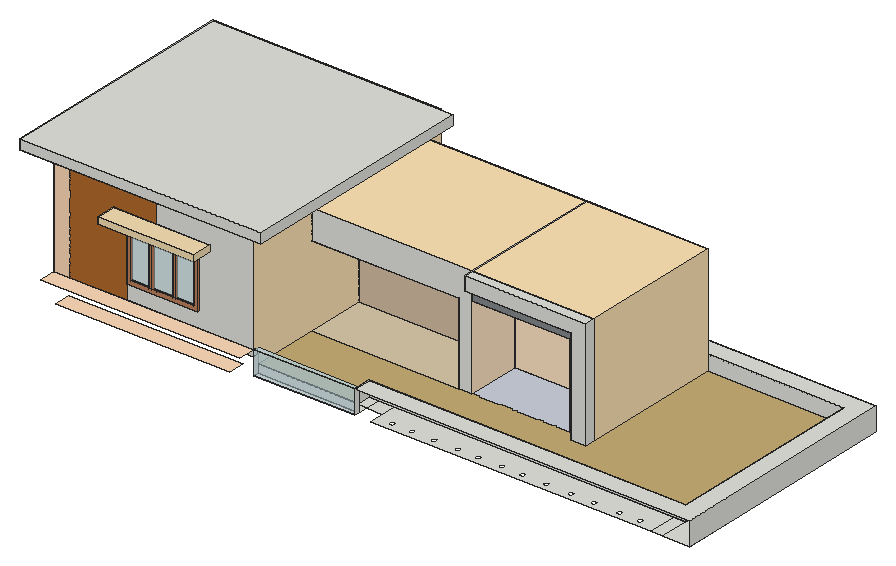
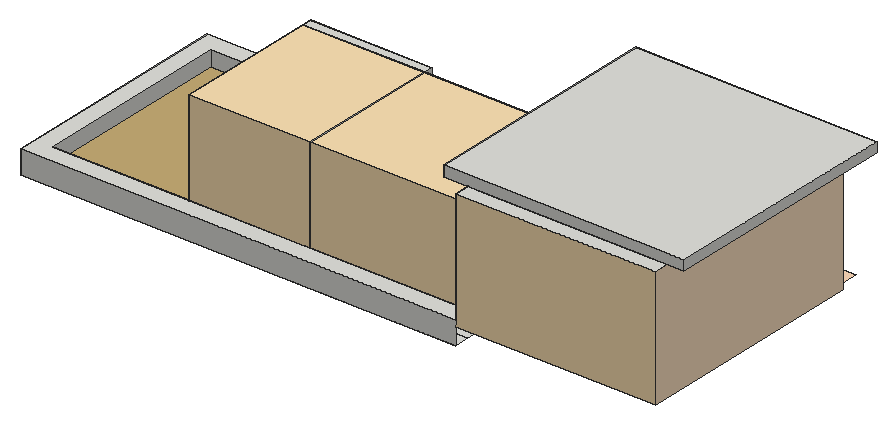
# SketchUp Ruby script. Lengths in inches.
U = 1.inch
M = Sketchup.active_model
def pt(a) = Geom::Point3d.new(a.map { |v| v * U })
def face(e, loops, mat)
  f = e.add_face(loops[0].map { |a| pt(a) })
  loops[1..].each { |l| e.add_face(l.map { |a| pt(a) }).erase! }
  f.material = f.back_material = mat if mat
  f
end
# faces: each face lists its corners as indices into pts; further lists are holes
def faces(e, pts, list, mat = nil) = list.each { |f| face(e, (f[0].is_a?(Array) ? f : [f]).map { |l| l.map { |i| pts[i] } }, mat) }
# xy, xz, yz: faces in a plane at the given z, y or x. An outline is a flat list of corners, or four numbers for a rectangle; further outlines are holes
def ring(l) = l.size == 4 ? [[l[0], l[1]], [l[2], l[1]], [l[2], l[3]], [l[0], l[3]]] : l.each_slice(2).to_a
def flat(e, list, mat, &to3) = list.each { |f| face(e, (f[0].is_a?(Array) ? f : [f]).map { |l| ring(l).map { |u, v| to3.(u, v) } }, mat) }
def xy(e, z, list, mat = nil) = flat(e, list, mat) { |x, y| [x, y, z] }
def xz(e, y, list, mat = nil) = flat(e, list, mat) { |x, z| [x, y, z] }
def yz(e, x, list, mat = nil) = flat(e, list, mat) { |y, z| [x, y, z] }
def lines(e, pts, list) = list.each { |a, b| e.add_line(pt(pts[a]), pt(pts[b])) }
# prism: a flat outline (further loops are holes) pulled along v
def prism(e, loops, v, mat = nil)
  f = face(e, loops, mat); d = Geom::Vector3d.new(v.map { |x| x * U })
  f.pushpull(f.normal.samedirection?(d) ? d.length : -d.length)
end
def box(e, o, s, mat = nil) = prism(e, [[o, [o[0] + s[0], o[1], o[2]], [o[0] + s[0], o[1] + s[1], o[2]], [o[0], o[1] + s[1], o[2]]]], [0, 0, s[2]], mat)
def at(x, y, z, deg = 0) = Geom::Transformation.translation(pt([x, y, z])) * Geom::Transformation.rotation(ORIGIN, Z_AXIS, deg.degrees)
def axes(o, x, y, z) = Geom::Transformation.new([*x, 0, *y, 0, *z, 0, *pt(o).to_a, 1])
def part(name) = M.definitions.add(name)
# library, detail: a bought-in or finely detailed component or shape, given as its bounding box
def library(name, o, s) = part(name).tap { |d| box(d.entities, o, s) }
def detail(e, o, s) = box(e.add_group.entities, o, s)
def put(e, d, t, mat = nil) = e.add_instance(d, t).tap { |i| i.material = mat if mat }
def group(e, t, mat = nil) = e.add_group.tap { |g| g.transformation = t; g.material = mat if mat }.entities
root = M.entities
M.materials.add("[0012_Bisque]").color = [255, 228, 196]
M.materials.add("[0027_PeachPuff]").color = [255, 218, 185]
M.materials.add("[0032_Moccasin]").color = [255, 228, 181]
M.materials.add("[0034_Wheat]").color = [245, 222, 179]
M.materials.add("[Blacktop Old 01]").color = [132, 136, 139]
M.materials.add("[Color M06]").color = [86, 86, 86]
M.materials.add("[Field Square Tile]").color = [217, 201, 169]
M.materials.add("[Formica Laminate Light]").color = [213, 189, 164]
M.materials.add("[Marble Carrara Floor Tile]").color = [204, 208, 219]
M.materials.add("[Tile Limestone Multi]").color = [199, 173, 118]
M.materials.add("[Translucent Glass Safety]").color = [204, 235, 244]
M.materials["[Translucent Glass Safety]"].alpha = 0.5
M.materials.add("[Wood Bamboo]").color = [177, 105, 43]
M.materials.add("[Wood Veneer 02]").color = [190, 128, 91]
c1 = library("Group\#1",[-0.5,-0.5,-0.1],[12.08,12.08,0.2])
c2 = library("Group\#2",[-0.5,-0.5,-0.1],[12.08,12.08,0.2])
c3 = library("Group\#3",[-0.5,-0.5,-0.1],[12.08,12.08,0.2])
c4 = library("Group\#4",[-0.5,-0.5,-0.1],[10.1875,10.1875,0.2])
c5 = library("Group\#5",[-0.5,-0.5,-0.1],[10.1875,10.1875,0.2])
c6 = library("Group\#6",[-0.5,-0.5,-0.1],[10.1875,10.1875,0.2])
c7 = library("Group\#7",[-0.5,-0.5,-0.1],[10.1875,10.1875,0.2])
c8 = library("Group\#8",[-0.5,-0.5,-0.1],[10.1875,10.1875,0.2])
c9 = library("Group\#9",[-0.5,-0.5,-0.1],[10.1875,10.1875,0.2])
xy(root,118.57,[[406.1,313.78,461.1,315.41]])
xy(root,129,[[272.73,223.85,374.48,229.35],[[391.12,223.85,391.12,315.41,461.1,315.41,461.1,311.53,526.2,311.53,526.2,315.41,684.44,315.41,684.44,458.94,711.13,458.94,711.13,223.85,684.44,223.85,684.44,268.03,671.95,268.03,671.95,223.85],[406,228.82,406.71,228.92,407.375,229.19,407.94,229.63,408.38,230.2,408.66,230.86,408.75,231.57,408.66,232.29,408.38,232.95,407.94,233.52,407.375,233.96,406.71,234.23,406,234.32,405.29,234.23,404.625,233.96,404.06,233.52,403.62,232.95,403.34,232.29,403.25,231.57,403.34,230.86,403.62,230.2,404.06,229.63,404.625,229.19,405.29,228.92],[426,228.82,426.71,228.92,427.375,229.19,427.94,229.63,428.38,230.2,428.66,230.86,428.75,231.57,428.66,232.29,428.38,232.95,427.94,233.52,427.375,233.96,426.71,234.23,426,234.32,425.29,234.23,424.625,233.96,424.06,233.52,423.62,232.95,423.34,232.29,423.25,231.57,423.34,230.86,423.62,230.2,424.06,229.63,424.625,229.19,425.29,228.92],[471.875,228.82,472.59,228.92,473.25,229.19,473.82,229.63,474.26,230.2,474.53,230.86,474.625,231.57,474.53,232.29,474.26,232.95,473.82,233.52,473.25,233.96,472.59,234.23,471.875,234.32,471.16,234.23,470.5,233.96,469.93,233.52,469.49,232.95,469.22,232.29,469.125,231.57,469.22,230.86,469.49,230.2,469.93,229.63,470.5,229.19,471.16,228.92],[492.8125,228.82,493.52,228.92,494.1875,229.19,494.76,229.63,495.19,230.2,495.47,230.86,495.5625,231.57,495.47,232.29,495.19,232.95,494.76,233.52,494.1875,233.96,493.52,234.23,492.8125,234.32,492.1,234.23,491.4375,233.96,490.87,233.52,490.43,232.95,490.16,232.29,490.0625,231.57,490.16,230.86,490.43,230.2,490.87,229.63,491.4375,229.19,492.1,228.92],[516.1875,228.82,516.9,228.92,517.5625,229.19,518.13,229.63,518.57,230.2,518.84,230.86,518.9375,231.57,518.84,232.29,518.57,232.95,518.13,233.52,517.5625,233.96,516.9,234.23,516.1875,234.32,515.48,234.23,514.8125,233.96,514.24,233.52,513.81,232.95,513.53,232.29,513.4375,231.57,513.53,230.86,513.81,230.2,514.24,229.63,514.8125,229.19,515.48,228.92],[537.375,228.82,538.09,228.92,538.75,229.19,539.32,229.63,539.76,230.2,540.03,230.86,540.125,231.57,540.03,232.29,539.76,232.95,539.32,233.52,538.75,233.96,538.09,234.23,537.375,234.32,536.66,234.23,536,233.96,535.43,233.52,534.99,232.95,534.72,232.29,534.625,231.57,534.72,230.86,534.99,230.2,535.43,229.63,536,229.19,536.66,228.92],[448.1875,228.82,448.9,228.92,449.5625,229.19,450.13,229.63,450.57,230.2,450.84,230.86,450.9375,231.57,450.84,232.29,450.57,232.95,450.13,233.52,449.5625,233.96,448.9,234.23,448.1875,234.32,447.48,234.23,446.8125,233.96,446.24,233.52,445.81,232.95,445.53,232.29,445.4375,231.57,445.53,230.86,445.81,230.2,446.24,229.63,446.8125,229.19,447.48,228.92],[561.125,228.82,561.84,228.92,562.5,229.19,563.07,229.63,563.51,230.2,563.78,230.86,563.875,231.57,563.78,232.29,563.51,232.95,563.07,233.52,562.5,233.96,561.84,234.23,561.125,234.32,560.41,234.23,559.75,233.96,559.18,233.52,558.74,232.95,558.47,232.29,558.375,231.57,558.47,230.86,558.74,230.2,559.18,229.63,559.75,229.19,560.41,228.92],[585.9375,228.82,586.65,228.92,587.3125,229.19,587.88,229.63,588.32,230.2,588.59,230.86,588.6875,231.57,588.59,232.29,588.32,232.95,587.88,233.52,587.3125,233.96,586.65,234.23,585.9375,234.32,585.23,234.23,584.5625,233.96,583.99,233.52,583.56,232.95,583.28,232.29,583.1875,231.57,583.28,230.86,583.56,230.2,583.99,229.63,584.5625,229.19,585.23,228.92],[609.0625,228.82,609.77,228.92,610.4375,229.19,611.01,229.63,611.44,230.2,611.72,230.86,611.8125,231.57,611.72,232.29,611.44,232.95,611.01,233.52,610.4375,233.96,609.77,234.23,609.0625,234.32,608.35,234.23,607.6875,233.96,607.12,233.52,606.68,232.95,606.41,232.29,606.3125,231.57,606.41,230.86,606.68,230.2,607.12,229.63,607.6875,229.19,608.35,228.92],[634.75,228.82,635.46,228.92,636.125,229.19,636.69,229.63,637.13,230.2,637.41,230.86,637.5,231.57,637.41,232.29,637.13,232.95,636.69,233.52,636.125,233.96,635.46,234.23,634.75,234.32,634.04,234.23,633.375,233.96,632.81,233.52,632.37,232.95,632.09,232.29,632,231.57,632.09,230.86,632.37,230.2,632.81,229.63,633.375,229.19,634.04,228.92],[655.5,228.82,656.21,228.92,656.875,229.19,657.44,229.63,657.88,230.2,658.16,230.86,658.25,231.57,658.16,232.29,657.88,232.95,657.44,233.52,656.875,233.96,656.21,234.23,655.5,234.32,654.79,234.23,654.125,233.96,653.56,233.52,653.12,232.95,652.84,232.29,652.75,231.57,652.84,230.86,653.12,230.2,653.56,229.63,654.125,229.19,654.79,228.92]],[671.95,223.85,684.44,268.03],[272.73,229.35,374.48,238.73],[272.73,238.73,374.48,315.41],
  [374.48,238.73,391.12,315.41],[461.1,311.53,526.2,315.41],[272.73,315.41,374.48,358.92],[374.48,315.41,391.12,358.92],[391.12,315.41,684.44,358.92],
  [272.73,358.92,374.48,444.0625],[374.48,358.92,391.12,444.0625],[391.12,358.92,668.6875,444.0625],[668.6875,358.92,684.44,458.94],[272.73,444.0625,374.48,458.94],
  [374.48,444.0625,391.12,458.94],[391.12,444.0625,668.6875,458.94]])
xy(root,135.55,[[87.11,206.91,261.95,223.85]],"[0027_PeachPuff]")
xy(root,137.125,[[540.98,287.63,556.35,297.19],[420.54,297.19,434.1,297.19,434.1,440.78,272.73,440.78,272.73,356.69,420.54,356.69],[531.85,297.19,556.35,297.19,556.35,440.78,434.1,440.78,434.1,351.13,531.85,351.13]])
xy(root,137.125,[[272.73,297.19,420.54,356.69]],"[Field Square Tile]")
xy(root,137.125,[[434.1,297.19,531.85,351.13]],"[Marble Carrara Floor Tile]")
xy(root,137.125,[[272.73,229.35,374.48,229.35,374.48,242,692.97,242,692.97,440.78,556.35,440.78,556.35,287.63,540.98,287.63,540.98,297.19,272.73,297.19]],"[Tile Limestone Multi]")
xy(root,146.125,[[87.11,238.73,261.95,444.0625]])
xy(root,152.4375,[[374.48,223.85,711.13,223.85,711.13,458.94,272.73,458.94,272.73,440.78,692.97,440.78,692.97,242,374.48,242]])
xy(root,152.4375,[[72.24,206.91,272.73,223.85]],"[0027_PeachPuff]")
xy(root,152.4375,[[272.73,223.85,374.48,229.35]],"[Translucent Glass Safety]")
xy(root,167.88,[[146.61,221.91,217.98,223.85]])
xy(root,171.94,[[169.08,221.91,172.21,223.85],[192.77,221.91,195.89,223.85]])
xy(root,171.94,[[150.67,221.91,169.08,223.85],[172.21,221.91,192.77,223.85],[195.89,221.91,213.92,223.85]],"[Wood Veneer 02]")
xy(root,218.58,[[272.73,297.19,420.54,356.69]],"[Wood Bamboo]")
xy(root,220.07,[[169.08,221.91,172.21,223.85],[192.77,221.91,195.89,223.85]])
xy(root,220.07,[[150.67,221.91,169.08,223.85],[172.21,221.91,192.77,223.85],[195.89,221.91,213.92,223.85]],"[Wood Veneer 02]")
xy(root,220.89,[[434.1,297.19,531.85,351.13]],"[Wood Bamboo]")
xy(root,224.13,[[146.61,221.91,217.98,223.85]],"[Wood Veneer 02]")
xy(root,224.89,[[131.94,203.66,228.51,223.85]],"[0034_Wheat]")
xy(root,231.27,[[131.94,203.66,228.51,223.85]],"[0034_Wheat]")
xy(root,233.8,[[434.1,287.63,540.98,297.19]])
xy(root,247.56,[[434.1,287.63,556.35,297.19]])
xy(root,247.56,[[272.73,297.19,434.1,440.78],[434.1,297.19,556.35,440.78]],"[0032_Moccasin]")
xy(root,266.125,[[72.24,223.85,272.73,238.73],[72.24,238.73,87.11,444.0625],[87.11,238.73,261.95,444.0625],[261.95,238.73,272.73,444.0625],[72.24,444.0625,272.73,458.94]])
xy(root,266.125,[[55.8,201.73,55.8,444.0625,72.24,444.0625,72.24,223.85,272.73,223.85,272.73,444.0625,297.48,444.0625,297.48,201.73]],"[Color M06]")
xy(root,276.1875,[[55.8,201.73,297.48,444.0625]])
xz(root,201.73,[[55.8,266.125,297.48,276.1875]])
xz(root,203.66,[[131.94,224.89,228.51,231.27]],"[0034_Wheat]")
xz(root,221.91,[[[146.61,167.88,217.98,224.13],[150.67,171.94,213.92,220.07]],[169.08,171.94,172.21,220.07],[192.77,171.94,195.89,220.07]],"[Wood Veneer 02]")
xz(root,223.85,[[72.24,146.125,272.73,152.4375],[146.61,152.4375,272.73,152.4375,272.73,256.625,175.77,256.625,175.77,231.27,228.51,231.27,228.51,224.89,175.91,224.89,175.91,224.13,217.98,224.13,217.98,167.88,146.61,167.88],[[146.61,167.88,217.98,224.13],[150.67,171.94,213.92,220.07]],[169.08,171.94,172.21,220.07],[192.77,171.94,195.89,220.07],
  [131.94,224.89,228.51,231.27]])
xz(root,223.85,[[72.24,152.4375,87.82,152.4375,87.82,256.625,272.73,256.625,272.73,266.125,72.24,266.125]],"[0027_PeachPuff]")
xz(root,223.85,[[272.73,129,374.48,152.4375],[150.67,171.94,169.08,220.07],[172.21,171.94,192.77,220.07],[195.89,171.94,213.92,220.07]],"[Translucent Glass Safety]")
xz(root,223.85,[[87.82,152.4375,146.61,152.4375,146.61,224.13,175.91,224.13,175.91,224.89,131.94,224.89,131.94,231.27,175.77,231.27,175.77,256.625,87.82,256.625]],"[Wood Bamboo]")
xz(root,229.35,[[272.73,129,374.48,137.125]])
xz(root,229.35,[[272.73,137.125,374.48,152.4375]],"[Translucent Glass Safety]")
xz(root,238.73,[[87.11,135.55,261.95,146.125],[87.11,146.125,261.95,266.125]])
xz(root,242,[[374.48,137.125,692.97,152.4375]])
xz(root,287.63,[[540.98,137.125,556.35,137.125,556.35,247.56,434.1,247.56,434.1,233.8,540.98,233.8]])
xz(root,297.19,[[420.54,137.125,434.1,137.125,434.1,247.56,272.73,247.56,272.73,218.58,420.54,218.58],[540.98,137.125,540.98,233.8,434.1,233.8,434.1,247.56,556.35,247.56,556.35,137.125]])
xz(root,297.19,[[531.85,137.125,540.98,137.125,540.98,233.8,434.1,233.8,434.1,220.89,531.85,220.89]],"[Blacktop Old 01]")
xz(root,351.13,[[434.1,137.125,531.85,220.89]],"[0012_Bisque]")
xz(root,356.69,[[272.73,137.125,420.54,218.58]],"[Formica Laminate Light]")
xz(root,440.78,[[272.73,137.125,434.1,152.4375],[434.1,137.125,556.35,152.4375],[556.35,137.125,692.97,152.4375]])
xz(root,440.78,[[272.73,152.4375,434.1,247.56],[434.1,152.4375,556.35,247.56]],"[0032_Moccasin]")
xz(root,444.0625,[[87.11,146.125,261.95,266.125],[55.8,266.125,297.48,276.1875]])
xz(root,458.94,[[272.73,129,711.13,152.4375]])
xz(root,458.94,[[72.24,146.125,272.73,266.125]],"[0032_Moccasin]")
yz(root,55.8,[[201.73,266.125,444.0625,276.1875]])
yz(root,72.24,[[223.85,146.125,458.94,266.125]],"[0012_Bisque]")
yz(root,87.11,[[238.73,146.125,444.0625,266.125]])
yz(root,131.94,[[203.66,224.89,223.85,231.27]],"[0034_Wheat]")
yz(root,146.61,[[221.91,167.88,223.85,224.13]],"[Wood Veneer 02]")
yz(root,150.67,[[221.91,171.94,223.85,220.07]],"[Wood Veneer 02]")
yz(root,169.08,[[221.91,171.94,223.85,220.07]],"[Wood Veneer 02]")
yz(root,172.21,[[221.91,171.94,223.85,220.07]],"[Wood Veneer 02]")
yz(root,192.77,[[221.91,171.94,223.85,220.07]],"[Wood Veneer 02]")
yz(root,195.89,[[221.91,171.94,223.85,220.07]],"[Wood Veneer 02]")
yz(root,213.92,[[221.91,171.94,223.85,220.07]],"[Wood Veneer 02]")
yz(root,217.98,[[221.91,167.88,223.85,224.13]],"[Wood Veneer 02]")
yz(root,228.51,[[203.66,224.89,223.85,231.27]],"[0034_Wheat]")
yz(root,261.95,[[238.73,146.125,444.0625,266.125]])
yz(root,272.73,[[223.85,129,229.35,146.125],[356.69,137.125,356.69,218.58,297.19,218.58,297.19,247.56,440.78,247.56,440.78,137.125],[223.85,146.125,229.35,152.4375]])
yz(root,272.73,[[229.35,137.125,356.69,137.125,356.69,218.58,297.19,218.58,297.19,247.56,440.78,247.56,440.78,152.4375,458.94,152.4375,458.94,266.125,223.85,266.125,223.85,152.4375,229.35,152.4375]],"[0032_Moccasin]")
yz(root,297.48,[[201.73,266.125,444.0625,276.1875]])
yz(root,374.48,[[223.85,129,229.35,152.4375],[229.35,137.125,242,152.4375]])
yz(root,420.54,[[297.19,137.125,356.69,218.58]],"[0012_Bisque]")
yz(root,434.1,[[351.13,137.125,351.13,220.89,297.19,220.89,297.19,247.56,440.78,247.56,440.78,137.125],[287.63,233.8,297.19,247.56]])
yz(root,434.1,[[297.19,137.125,351.13,220.89]],"[0012_Bisque]")
yz(root,531.85,[[297.19,137.125,351.13,220.89]],"[0012_Bisque]")
yz(root,540.98,[[287.63,137.125,297.19,233.8]])
yz(root,556.35,[[287.63,137.125,297.19,247.56]])
yz(root,556.35,[[297.19,137.125,440.78,247.56]],"[0032_Moccasin]")
yz(root,692.97,[[242,137.125,440.78,152.4375]])
yz(root,711.13,[[223.85,129,458.94,152.4375]])
put(root,c1,axes([290.77,305.76,218.58],[-1,0,0],[0,1,0],[0,0,-1]))
put(root,c2,axes([346.96,305.76,218.58],[-1,0,0],[0,1,0],[0,0,-1]))
put(root,c3,axes([408.09,305.76,218.58],[-1,0,0],[0,1,0],[0,0,-1]))
put(root,c4,axes([460.45,301.68,220.89],[-1,0,0],[0,1,0],[0,0,-1]))
put(root,c5,axes([460.45,319.12,220.89],[-1,0,0],[0,1,0],[0,0,-1]))
put(root,c6,axes([460.45,337.55,220.89],[-1,0,0],[0,1,0],[0,0,-1]))
put(root,c7,axes([518.01,301.68,220.89],[-1,0,0],[0,1,0],[0,0,-1]))
put(root,c8,axes([518.01,319.37,220.89],[-1,0,0],[0,1,0],[0,0,-1]))
put(root,c9,axes([518.01,335.37,220.89],[-1,0,0],[0,1,0],[0,0,-1]))
